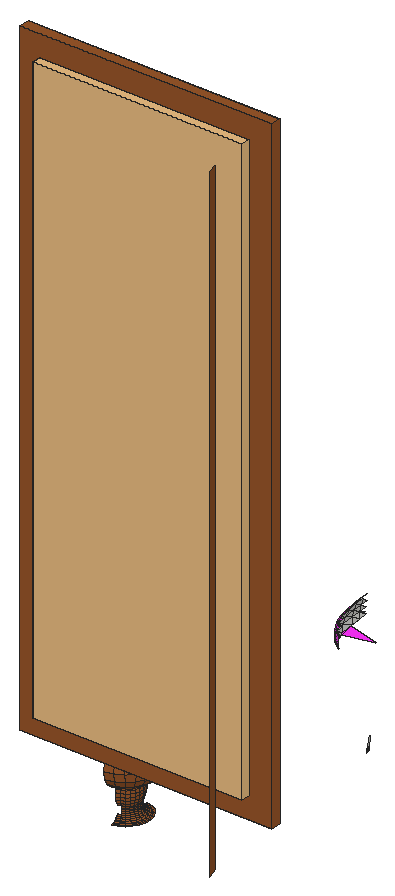
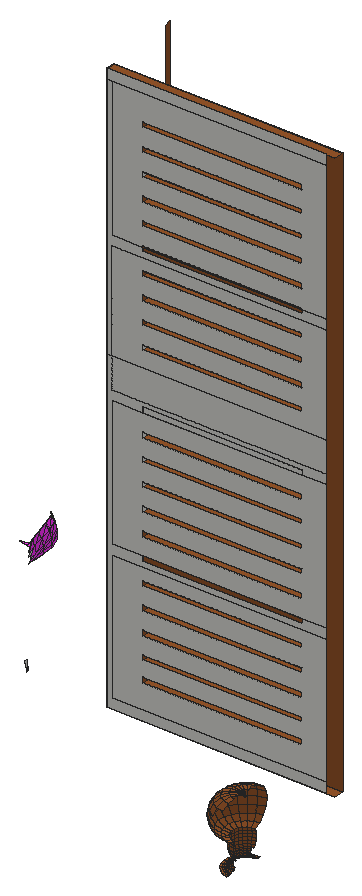
# SketchUp Ruby script. Lengths in inches.
U = 1.inch
M = Sketchup.active_model
def pt(a) = Geom::Point3d.new(a.map { |v| v * U })
def face(e, loops, mat)
  f = e.add_face(loops[0].map { |a| pt(a) })
  loops[1..].each { |l| e.add_face(l.map { |a| pt(a) }).erase! }
  f.material = f.back_material = mat if mat
  f
end
# faces: each face lists its corners as indices into pts; further lists are holes
def faces(e, pts, list, mat = nil) = list.each { |f| face(e, (f[0].is_a?(Array) ? f : [f]).map { |l| l.map { |i| pts[i] } }, mat) }
# xy, xz, yz: faces in a plane at the given z, y or x. An outline is a flat list of corners, or four numbers for a rectangle; further outlines are holes
def ring(l) = l.size == 4 ? [[l[0], l[1]], [l[2], l[1]], [l[2], l[3]], [l[0], l[3]]] : l.each_slice(2).to_a
def flat(e, list, mat, &to3) = list.each { |f| face(e, (f[0].is_a?(Array) ? f : [f]).map { |l| ring(l).map { |u, v| to3.(u, v) } }, mat) }
def xy(e, z, list, mat = nil) = flat(e, list, mat) { |x, y| [x, y, z] }
def xz(e, y, list, mat = nil) = flat(e, list, mat) { |x, z| [x, y, z] }
def yz(e, x, list, mat = nil) = flat(e, list, mat) { |y, z| [x, y, z] }
def lines(e, pts, list) = list.each { |a, b| e.add_line(pt(pts[a]), pt(pts[b])) }
# prism: a flat outline (further loops are holes) pulled along v
def prism(e, loops, v, mat = nil)
  f = face(e, loops, mat); d = Geom::Vector3d.new(v.map { |x| x * U })
  f.pushpull(f.normal.samedirection?(d) ? d.length : -d.length)
end
def box(e, o, s, mat = nil) = prism(e, [[o, [o[0] + s[0], o[1], o[2]], [o[0] + s[0], o[1] + s[1], o[2]], [o[0], o[1] + s[1], o[2]]]], [0, 0, s[2]], mat)
def at(x, y, z, deg = 0) = Geom::Transformation.translation(pt([x, y, z])) * Geom::Transformation.rotation(ORIGIN, Z_AXIS, deg.degrees)
def axes(o, x, y, z) = Geom::Transformation.new([*x, 0, *y, 0, *z, 0, *pt(o).to_a, 1])
def part(name) = M.definitions.add(name)
# library, detail: a bought-in or finely detailed component or shape, given as its bounding box
def library(name, o, s) = part(name).tap { |d| box(d.entities, o, s) }
def detail(e, o, s) = box(e.add_group.entities, o, s)
def put(e, d, t, mat = nil) = e.add_instance(d, t).tap { |i| i.material = mat if mat }
def group(e, t, mat = nil) = e.add_group.tap { |g| g.transformation = t; g.material = mat if mat }.entities
root = M.entities
M.materials.add("[Color K04]").color = [255, 50, 255]
M.materials.add("[Wood Cherry Original]").color = [152, 86, 42]
c1 = part("Group\#13")
detail(c1.entities,[0,0,0],[19.875,0.8125,55.92])
xy(root,6,[[161.3,47.97,161.84,48.11,161.78,48.25,161.28,48.12],[161.84,48.11,162.32,48.39,162.23,48.51,161.78,48.25],[162.32,48.39,162.72,48.78,162.6,48.87,162.23,48.51],[162.72,48.78,163,49.26,162.86,49.32,162.6,48.87],[163,49.26,163.15,49.8,163,49.82,162.86,49.32],
  [163.15,49.8,163.15,50.36,163,50.34,163,49.82],[163,50.34,163.15,50.36,163.01,50.9,162.87,50.84],[162.87,50.84,163.01,50.9,162.73,51.38,162.61,51.29],[162.61,51.29,162.73,51.38,162.34,51.78,162.24,51.66],[162.24,51.66,162.34,51.78,161.85,52.06,161.8,51.92],
  [161.8,51.92,161.85,52.06,161.32,52.21,161.3,52.06]],"[Wood Cherry Original]")
xy(root,13.08,[[154.9,45.11,178.85,46.11]],"[Wood Cherry Original]")
xy(root,16.73,[[158.4,45.11,175.02,46.11]],"[Wood Cherry Original]")
xy(root,17.26,[[158.4,45.11,175.02,46.11]],"[Wood Cherry Original]")
xy(root,18.83,[[158.4,45.11,175.02,46.11]],"[Wood Cherry Original]")
xy(root,19.33,[[158.4,45.11,175.02,46.11]],"[Wood Cherry Original]")
xy(root,21.15,[[158.4,45.11,175.02,46.11]],"[Wood Cherry Original]")
xy(root,21.65,[[158.4,45.11,175.02,46.11]],"[Wood Cherry Original]")
xy(root,23.48,[[158.4,45.11,175.02,46.11]],"[Wood Cherry Original]")
xy(root,23.98,[[158.4,45.11,175.02,46.11]],"[Wood Cherry Original]")
xy(root,25.8,[[158.4,45.11,175.02,46.11]],"[Wood Cherry Original]")
xy(root,26.3,[[158.4,45.11,175.02,46.11]],"[Wood Cherry Original]")
xy(root,28.125,[[158.4,45.11,175.02,46.11]],"[Wood Cherry Original]")
xy(root,28.625,[[158.4,45.11,175.02,46.11]],"[Wood Cherry Original]")
xy(root,30.45,[[158.4,45.11,175.02,46.11]],"[Wood Cherry Original]")
xy(root,30.95,[[158.4,45.11,175.02,46.11]],"[Wood Cherry Original]")
xy(root,32.78,[[158.4,45.11,175.02,46.11]],"[Wood Cherry Original]")
xy(root,33.28,[[158.4,45.11,175.02,46.11]],"[Wood Cherry Original]")
xy(root,35.1,[[158.4,45.11,175.02,46.11]],"[Wood Cherry Original]")
xy(root,35.6,[[158.4,45.11,175.02,46.11]])
xy(root,37.43,[[158.4,45.11,175.02,46.11]],"[Wood Cherry Original]")
xy(root,37.93,[[158.4,45.11,175.02,46.11]])
xy(root,39.75,[[158.4,45.11,175.02,46.11]],"[Wood Cherry Original]")
xy(root,40.25,[[158.4,45.11,175.02,46.11]])
xy(root,42.08,[[158.4,45.11,175.02,46.11]],"[Wood Cherry Original]")
xy(root,42.58,[[158.4,45.11,175.02,46.11]])
xy(root,47.97,[[158.4,45.11,175.02,46.11]],"[Wood Cherry Original]")
xy(root,48.47,[[158.4,45.11,175.02,46.11]])
xy(root,50.29,[[158.4,45.11,175.02,46.11]],"[Wood Cherry Original]")
xy(root,50.79,[[158.4,45.11,175.02,46.11]],"[Wood Cherry Original]")
xy(root,52.62,[[158.4,45.11,175.02,46.11]],"[Wood Cherry Original]")
xy(root,53.12,[[158.4,45.11,175.02,46.11]],"[Wood Cherry Original]")
xy(root,54.94,[[158.4,45.11,175.02,46.11]],"[Wood Cherry Original]")
xy(root,55.44,[[158.4,45.11,175.02,46.11]],"[Wood Cherry Original]")
xy(root,57.27,[[158.4,45.11,175.02,46.11]],"[Wood Cherry Original]")
xy(root,57.77,[[158.4,45.11,175.02,46.11]],"[Wood Cherry Original]")
xy(root,59.59,[[158.4,45.11,175.02,46.11]],"[Wood Cherry Original]")
xy(root,60.09,[[158.4,45.11,175.02,46.11]],"[Wood Cherry Original]")
xy(root,61.92,[[158.4,45.11,175.02,46.11]],"[Wood Cherry Original]")
xy(root,62.42,[[158.4,45.11,175.02,46.11]],"[Wood Cherry Original]")
xy(root,64.24,[[158.4,45.11,175.02,46.11]],"[Wood Cherry Original]")
xy(root,64.74,[[158.4,45.11,175.02,46.11]])
xy(root,66.57,[[158.4,45.11,175.02,46.11]],"[Wood Cherry Original]")
xy(root,67.07,[[158.4,45.11,175.02,46.11]])
xy(root,68.89,[[158.4,45.11,175.02,46.11]],"[Wood Cherry Original]")
xy(root,69.39,[[158.4,45.11,175.02,46.11]])
xy(root,73.08,[[154.9,45.11,178.85,46.11]],"[Wood Cherry Original]")
xz(root,45.11,[[[154.9,13.08,178.85,73.08],[158.4,16.73,175.02,69.39]],[158.4,17.26,175.02,18.83],[158.4,19.33,175.02,21.15],[158.4,21.65,175.02,23.48],[158.4,23.98,175.02,25.8],
  [158.4,26.3,175.02,28.125],[158.4,28.625,175.02,30.45],[158.4,30.95,175.02,32.78],[158.4,33.28,175.02,35.1],[158.4,35.6,175.02,37.43],
  [158.4,37.93,175.02,39.75],[158.4,40.25,175.02,42.08],[158.4,42.58,175.02,47.97],[158.4,48.47,175.02,50.29],[158.4,50.79,175.02,52.62],
  [158.4,53.12,175.02,54.94],[158.4,55.44,175.02,57.27],[158.4,57.77,175.02,59.59],[158.4,60.09,175.02,61.92],[158.4,62.42,175.02,64.24],
  [158.4,64.74,175.02,66.57],[158.4,67.07,175.02,68.89]],"[Wood Cherry Original]")
xz(root,46.11,[[155.9,13.08,178.85,13.08,178.85,46.26,178.35,46.26,178.35,43.08,155.9,43.08,155.9,42.08,158.4,42.08,158.4,42.58,175.02,42.58,175.02,42.08,178.35,42.08,178.35,28.58,175.02,28.58,175.02,28.125,158.4,28.125,158.4,28.58,155.9,28.58,155.9,27.58,178.35,27.58,178.35,14.08,155.9,14.08],[[155.9,13.08,155.9,43.08,178.35,43.08,178.35,46.26,178.85,46.26,178.85,13.08],[158.4,16.73,175.02,17.26],[158.4,42.08,175.02,42.58],[158.4,39.75,175.02,40.25],[158.4,37.43,175.02,37.93],[158.4,35.1,175.02,35.6],[158.4,32.78,175.02,33.28],[158.4,30.45,175.02,30.95],[158.4,28.125,175.02,28.625],[158.4,25.8,175.02,26.3],[158.4,23.48,175.02,23.98],[158.4,18.83,175.02,19.33],[158.4,21.15,175.02,21.65]],[158.4,42.08,175.02,42.58],[155.9,43.08,178.35,46.26],[178.35,46.26,178.85,46.26,178.85,72.08,178.35,72.08,178.35,57.58,175.02,57.58,175.02,57.27,158.4,57.27,158.4,57.58,155.9,57.58,155.9,56.58,178.35,56.58],
  [[155.9,46.26,178.35,56.58],[158.4,47.97,175.02,48.47],[158.4,50.29,175.02,50.79],[158.4,52.62,175.02,53.12],[158.4,54.94,175.02,55.44]],[[178.35,46.26,178.35,56.58,155.9,56.58,155.9,72.08,178.85,72.08,178.85,46.26],[158.4,68.89,175.02,69.39],[158.4,66.57,175.02,67.07],[158.4,64.24,175.02,64.74],[158.4,61.92,175.02,62.42],[158.4,59.59,175.02,60.09],[158.4,57.27,175.02,57.77]],[155.9,72.08,178.85,73.08]])
xz(root,46.11,[[158.4,28.125,175.02,28.58],[158.4,57.27,175.02,57.58]],"[Wood Cherry Original]")
yz(root,162.22,[[49.93,6.79,50.24,6.94]],"[Wood Cherry Original]")
yz(root,175.02,[[45.11,32.78,46.11,33.28],[45.11,35.1,46.11,35.6],[45.11,37.43,46.11,37.93],[45.11,39.75,46.11,40.25],[45.11,42.08,46.11,42.58],
  [45.11,47.97,46.11,48.47],[45.11,64.24,46.11,64.74]])
yz(root,175.02,[[45.11,16.73,46.11,17.26],[45.11,18.83,46.11,19.33],[45.11,21.15,46.11,21.65],[45.11,23.48,46.11,23.98],[45.11,25.8,46.11,26.3],
  [45.11,28.125,46.11,28.625],[45.11,30.45,46.11,30.95],[45.11,50.29,46.11,50.79],[45.11,52.62,46.11,53.12],[45.11,54.94,46.11,55.44],
  [45.11,57.27,46.11,57.77],[45.11,59.59,46.11,60.09],[45.11,61.92,46.11,62.42],[45.11,66.57,46.11,67.07],[45.11,68.89,46.11,69.39]],"[Wood Cherry Original]")
yz(root,178.85,[[45.11,13.08,46.11,73.08]],"[Wood Cherry Original]")
p = [[161.26,48.26,6.03],[161.28,48.12,6],[161.78,48.25,6],[161.73,48.39,6.03],[162.23,48.51,6],[162.14,48.625,6.03],
  [161.24,48.4,6.08],[161.67,48.52,6.08],[162.06,48.74,6.08],[162.6,48.87,6],[162.48,48.96,6.03],[162.37,49.05,6.08],
  [162.86,49.32,6],[162.72,49.375,6.03],[162.59,49.43,6.08],[163,49.82,6],[162.85,49.84,6.03],[162.71,49.86,6.08],
  [162.85,50.32,6.03],[162.71,50.3,6.08],[163,50.34,6],[162.73,50.78,6.03],[162.6,50.73,6.08],[162.87,50.84,6],
  [162.49,51.2,6.03],[162.38,51.11,6.08],[162.61,51.29,6],[162.15,51.54,6.03],[162.07,51.43,6.08],[162.24,51.66,6],
  [161.74,51.78,6.03],[161.68,51.65,6.08],[161.8,51.92,6],[161.28,51.91,6.03],[161.26,51.77,6.08],[161.3,52.06,6],
  [161.23,48.53,6.16],[161.62,48.64,6.16],[161.98,48.84,6.16],[162.27,49.13,6.16],[162.47,49.48,6.16],[162.58,49.875,6.16],
  [162.58,50.29,6.16],[162.48,50.68,6.16],[162.27,51.04,6.16],[161.99,51.33,6.16],[161.63,51.53,6.16],[161.24,51.64,6.16],
  [161.21,48.65,6.25],[161.58,48.74,6.25],[161.91,48.93,6.25],[162.18,49.2,6.25],[162.37,49.53,6.25],[162.47,49.89,6.25],
  [162.47,50.27,6.25],[162.37,50.64,6.25],[162.18,50.97,6.25],[161.92,51.23,6.25],[161.59,51.43,6.25],[161.22,51.52,6.25],
  [161.2,48.74,6.37],[161.54,48.83,6.37],[161.85,49.01,6.37],[162.1,49.26,6.37],[162.28,49.5625,6.37],[162.37,49.91,6.37],
  [162.37,50.26,6.37],[162.28,50.6,6.37],[162.11,50.91,6.37],[161.86,51.16,6.37],[161.55,51.34,6.37],[161.21,51.43,6.37],
  [161.19,48.82,6.5],[161.51,48.9,6.5],[161.8,49.07,6.5],[162.04,49.3,6.5],[162.21,49.59,6.5],[162.3,49.92,6.5],
  [162.3,50.25,6.5],[162.21,50.57,6.5],[162.05,50.86,6.5],[161.8125,51.1,6.5],[161.52,51.27,6.5],[161.2,51.35,6.5],
  [161.49,48.95,6.64],[161.77,49.11,6.64],[162,49.34,6.64],[162.16,49.61,6.64],[162.24,49.92,6.64],[162.25,50.24,6.64],
  [162.16,50.55,6.64],[162,50.83,6.64],[161.78,51.06,6.64],[161.5,51.22,6.64],[161.48,48.98,6.79],[161.76,49.13,6.79],
  [161.98,49.35,6.79],[162.14,49.62,6.79],[162.22,49.93,6.79],[162.22,50.24,6.79],[162.14,50.54,6.79],[161.98,50.82,6.79],
  [161.76,51.04,6.79],[161.49,51.2,6.79],[161.48,48.97,6.94],[161.76,49.13,6.94],[161.98,49.35,6.94],[162.14,49.62,6.94],
  [162.22,49.93,6.94],[162.22,50.24,6.94],[162.14,50.54,6.94],[161.98,50.82,6.94],[161.76,51.04,6.94],[161.49,51.2,6.94],
  [161.49,48.95,7.09],[161.77,49.11,7.09],[162,49.34,7.09],[162.16,49.61,7.09],[162.25,49.92,7.09],[162.25,50.24,7.09],
  [162.16,50.55,7.09],[162.01,50.83,7.09],[161.78,51.06,7.09],[161.5,51.22,7.09],[161.51,48.9,7.23],[161.8,49.07,7.23],
  [162.04,49.3,7.23],[162.21,49.59,7.23],[162.3,49.92,7.23],[162.3,50.25,7.23],[162.21,50.57,7.23],[162.05,50.86,7.23],
  [161.8125,51.1,7.23],[161.52,51.27,7.23],[161.19,51.3,7.09],[161.2,51.36,7.23],[161.2,48.71,7.51],[161.19,48.82,7.23],
  [161.56,48.8,7.51],[161.87,48.98,7.51],[162.13,49.24,7.51],[162.3125,49.55,7.51],[162.41,49.9,7.51],[162.41,50.26,7.51],
  [162.32,50.61,7.51],[162.14,50.93,7.51],[161.88,51.1875,7.51],[161.57,51.37,7.51],[161.22,51.47,7.51],[161.21,48.63,7.8],
  [161.58,48.73,7.8],[161.92,48.92,7.8],[162.1875,49.1875,7.8],[162.38,49.52,7.8],[162.48,49.89,7.8],[162.48,50.27,7.8],
  [162.39,50.64,7.8],[162.2,50.98,7.8],[161.93,51.25,7.8],[161.59,51.44,7.8],[161.23,51.54,7.8],[161.22,48.59,8.1],
  [161.6,48.69,8.1],[161.94,48.89,8.1],[162.22,49.16,8.1],[162.42,49.5,8.1],[162.52,49.88,8.1],[162.52,50.28,8.1],
  [162.42,50.66,8.1],[162.23,51,8.1],[161.95,51.28,8.1],[161.61,51.48,8.1],[161.23,51.58,8.1],[161.22,48.59,8.4],
  [161.6,48.69,8.4],[161.94,48.89,8.4],[162.22,49.16,8.4],[162.42,49.5,8.4],[162.52,49.88,8.4],[162.53,50.28,8.4],
  [162.43,50.66,8.4],[162.23,51,8.4],[161.95,51.28,8.4],[161.61,51.48,8.4],[161.23,51.58,8.4],[161.22,48.62,8.7],
  [161.59,48.72,8.7],[161.92,48.91,8.7],[162.2,49.18,8.7],[162.39,49.52,8.7],[162.49,49.89,8.7],[162.49,50.27,8.7],
  [162.39,50.65,8.7],[162.2,50.98,8.7],[161.93,51.25,8.7],[161.6,51.45,8.7],[161.23,51.55,8.7],[161.21,48.69,8.99],
  [161.5625,48.79,8.99],[161.88,48.97,8.99],[162.14,49.23,8.99],[162.32,49.54,8.99],[162.42,49.9,8.99],[162.42,50.27,8.99],
  [162.33,50.62,8.99],[162.15,50.9375,8.99],[161.89,51.2,8.99],[161.57,51.38,8.99],[161.22,51.48,8.99],[161.3,48,9.21],
  [161.83,48.14,9.21],[162.3,48.41,9.21],[162.7,48.8,9.21],[162.97,49.27,9.21],[163.12,49.8,9.21],[163.12,50.35,9.21],
  [162.98,50.89,9.21],[162.71,51.36,9.21],[162.32,51.75,9.21],[161.84,52.03,9.21],[161.3125,52.18,9.21],[161.37,47.42,9.66],
  [162.05,47.6,9.66],[162.66,47.95,9.66],[163.15,48.44,9.66],[163.51,49.05,9.66],[163.69,49.73,9.66],[163.69,50.43,9.66],
  [163.51,51.11,9.66],[163.17,51.71,9.66],[162.67,52.21,9.66],[162.07,52.57,9.66],[161.39,52.75,9.66],[161.42,47.04,10.28],
  [162.19,47.25,10.28],[162.89,47.65,10.28],[163.45,48.21,10.28],[163.86,48.9,10.28],[164.07,49.68,10.28],[164.07,50.48,10.28],
  [163.87,51.25,10.28],[163.47,51.94,10.28],[162.9,52.51,10.28],[162.21,52.92,10.28],[161.43,46.91,11],[162.24,47.125,11],
  [162.97,47.54,11],[163.56,48.13,11],[163.98,48.85,11],[164.2,49.66,11],[164.2,50.49,11],[163.99,51.3,11],
  [163.57,52.03,11],[162.99,52.62,11],[161.42,47.04,11.72],[162.19,47.25,11.72],[162.89,47.65,11.72],[163.45,48.21,11.72],
  [163.86,48.9,11.72],[164.07,49.68,11.72],[164.07,50.48,11.72],[163.87,51.25,11.72],[163.47,51.94,11.72],[162.9,52.51,11.72],
  [161.37,47.42,12.34],[162.05,47.6,12.34],[162.66,47.95,12.34],[163.15,48.44,12.34],[163.51,49.05,12.34],[163.69,49.73,12.34],
  [163.69,50.43,12.34],[163.51,51.11,12.34],[163.17,51.71,12.34],[162.67,52.21,12.34],[162.21,52.92,11.72],[162.07,52.57,12.34],
  [161.3,48,12.79],[161.83,48.14,12.79],[162.3,48.41,12.79],[162.7,48.8,12.79],[162.97,49.27,12.79],[163.12,49.8,12.79],
  [163.12,50.35,12.79],[162.98,50.89,12.79],[162.71,51.36,12.79],[162.32,51.75,12.79],[161.84,52.03,12.79],[161.39,52.75,12.34],
  [161.3125,52.18,12.79],[161.03,50.09,12.67],[161.56,49.68,12.97],[161.65,49.83,12.97],[161.69,50,12.97],[161.69,50.17,12.97],
  [161.65,50.34,12.97],[161.5625,50.49,12.97],[161.21,48.69,13.01],[161.5625,48.79,13.01],[161.88,48.97,13.01],[162.14,49.23,13.01],
  [162.32,49.54,13.01],[162.42,49.9,13.01],[162.42,50.27,13.01],[162.33,50.62,13.01],[162.15,50.9375,13.01],[161.89,51.2,13.01],
  [161.57,51.38,13.01],[161.22,51.48,13.01],[161.28,49.47,12.97],[161.43,49.55,12.97],[161.4375,50.62,12.97],[161.29,50.71,12.97],
  [179.45,37.53,13.08],[179.8,36.6,13.08],[179.8,36.6,73.08],[179.45,37.53,73.08],[179.45,37.53,46.26],[182.43,51.92,17.77],
  [182.35,52.19,17.8125],[182.35,52.2,17.86],[182.4,52.07,18],[182.44,51.93,18.14],[182.34,52.25,17.82],[182.35,52.24,18.01],
  [182.3,52.48,18.99],[182.4,52.09,18.17],[182.4,52.16,18.88],[182.35,52.23,18.19],[182.13,48.48,28.67],[182.22,48.5,28.59],
  [182.89,47.98,28.59],[181.67,49.76,28.67],[181.75,49.77,28.59],[181.58,51.11,28.65],[181.5,51.1,28.73],[184.52,50.36,28.59],
  [182.13,48.48,28.96],[182.87,47.89,28.67],[182.87,47.89,28.96],[182.27,48.54,28.72],[182.26,48.59,29.63],[182.9,48.03,29.63],
  [181.67,49.76,28.96],[181.81,49.78,28.72],[181.79,49.8125,29.53],[181.5,51.1,28.96],[181.63,51.12,28.78],[181.375,52.2,28.96],
  [181.375,52.2,28.74],[181.45,52.22,28.66],[181.48,52.21,29.37],[181.51,52.23,28.79],[181.39,53.13,28.71],[181.625,51.09,29.45],
  [181.26,53.1,28.875],[181.49,51.08,29.47],[181.34,52.1875,29.38],[182.86,47.9,29.65],[182.14,48.51,29.65],[181.66,49.78,29.55],
  [181.23,53.09,29.34],[181.45,52.23,29.97],[181.59,52.25,29.9375],[181.37,53.11,29.33],[181.64,51.15,30.09],[181.77,51.17,30.05],
  [182.38,48.68,30.28],[181.98,49.86,30.17],[181.85,49.83,30.23],[182.9,48.04,30.32],[182.27,48.6,30.32],[182.93,48.17,30.28],
  [181.93,51.25,30.58],[181.72,52.32,30.46],[181.3,53.11,29.89],[181.6,52.3,30.55],[181.4375,53.13,29.86],[181.82,51.23,30.68],
  [182.16,49.97,30.79],[182.25,49.98,30.67],[182.51,48.74,30.9],[182.6,48.79,30.78],[182.93,48.29,30.9],[181.9,51.25,30.66],
  [181.67,52.3125,30.53],[181.47,53.14,30.46],[182.23,49.98,30.75],[182.58,48.78,30.86]]
faces(root,p,[[0,1,2,3],[3,2,4,5],[6,0,3,7],[7,3,5,8],[5,4,9,10],[8,5,10,11],[10,9,12,13],[11,10,13,14],
  [13,12,15,16],[14,13,16,17],[17,16,18,19],[16,15,20,18],[19,18,21,22],[18,20,23,21],[22,21,24,25],[21,23,26,24],
  [25,24,27,28],[24,26,29,27],[28,27,30,31],[27,29,32,30],[31,30,33,34],[30,32,35,33],[36,6,7,37],[37,7,8,38],
  [38,8,11,39],[39,11,14,40],[40,14,17,41],[41,17,19,42],[42,19,22,43],[43,22,25,44],[44,25,28,45],[45,28,31,46],
  [46,31,34,47],[48,36,37,49],[49,37,38,50],[50,38,39,51],[51,39,40,52],[52,40,41,53],[53,41,42,54],[54,42,43,55],
  [55,43,44,56],[56,44,45,57],[57,45,46,58],[58,46,47,59],[60,48,49,61],[61,49,50,62],[62,50,51,63],[63,51,52,64],
  [64,52,53,65],[65,53,54,66],[66,54,55,67],[67,55,56,68],[68,56,57,69],[69,57,58,70],[70,58,59,71],[72,60,61,73],
  [73,61,62,74],[74,62,63,75],[75,63,64,76],[76,64,65,77],[77,65,66,78],[78,66,67,79],[79,67,68,80],[80,68,69,81],
  [81,69,70,82],[82,70,71,83],[84,73,74,85],[85,74,75,86],[86,75,76,87],[87,76,77,88],[88,77,78,89],[89,78,79,90],
  [90,79,80,91],[91,80,81,92],[92,81,82,93],[94,84,85,95],[95,85,86,96],[96,86,87,97],[97,87,88,98],[98,88,89,99],
  [99,89,90,100],[100,90,91,101],[101,91,92,102],[102,92,93,103],[104,94,95,105],[105,95,96,106],[106,96,97,107],[107,97,98,108],
  [109,99,100,110],[110,100,101,111],[111,101,102,112],[112,102,103,113],[114,104,105,115],[115,105,106,116],[116,106,107,117],[117,107,108,118],
  [118,108,109,119],[119,109,110,120],[120,110,111,121],[121,111,112,122],[122,112,113,123],[124,114,115,125],[125,115,116,126],[126,116,117,127],
  [127,117,118,128],[128,118,119,129],[129,119,120,130],[130,120,121,131],[131,121,122,132],[132,122,123,133],[133,123,134,135],[136,137,124,138],
  [138,124,125,139],[139,125,126,140],[140,126,127,141],[141,127,128,142],[142,128,129,143],[143,129,130,144],[144,130,131,145],[145,131,132,146],
  [146,132,133,147],[147,133,135,148],[149,136,138,150],[150,138,139,151],[151,139,140,152],[152,140,141,153],[153,141,142,154],[154,142,143,155],
  [155,143,144,156],[156,144,145,157],[157,145,146,158],[158,146,147,159],[159,147,148,160],[161,149,150,162],[162,150,151,163],[163,151,152,164],
  [164,152,153,165],[165,153,154,166],[166,154,155,167],[167,155,156,168],[168,156,157,169],[169,157,158,170],[170,158,159,171],[171,159,160,172],
  [173,161,162,174],[174,162,163,175],[175,163,164,176],[176,164,165,177],[177,165,166,178],[178,166,167,179],[179,167,168,180],[180,168,169,181],
  [181,169,170,182],[182,170,171,183],[183,171,172,184],[185,173,174,186],[186,174,175,187],[187,175,176,188],[188,176,177,189],[189,177,178,190],
  [190,178,179,191],[191,179,180,192],[192,180,181,193],[193,181,182,194],[194,182,183,195],[195,183,184,196],[197,185,186,198],[198,186,187,199],
  [199,187,188,200],[200,188,189,201],[201,189,190,202],[202,190,191,203],[203,191,192,204],[204,192,193,205],[205,193,194,206],[206,194,195,207],
  [207,195,196,208],[209,197,198,210],[210,198,199,211],[211,199,200,212],[212,200,201,213],[213,201,202,214],[214,202,203,215],[215,203,204,216],
  [216,204,205,217],[217,205,206,218],[218,206,207,219],[219,207,208,220],[221,209,210,222],[222,210,211,223],[223,211,212,224],[224,212,213,225],
  [225,213,214,226],[226,214,215,227],[227,215,216,228],[228,216,217,229],[229,217,218,230],[230,218,219,231],[231,219,220,232],[233,221,222,234],
  [234,222,223,235],[235,223,224,236],[236,224,225,237],[237,225,226,238],[238,226,227,239],[239,227,228,240],[240,228,229,241],[241,229,230,242],
  [242,230,231,243],[244,233,234,245],[245,234,235,246],[246,235,236,247],[247,236,237,248],[248,237,238,249],[249,238,239,250],[250,239,240,251],
  [251,240,241,252],[252,241,242,253],[254,244,245,255],[255,245,246,256],[256,246,247,257],[257,247,248,258],[258,248,249,259],[259,249,250,260],
  [260,250,251,261],[261,251,252,262],[262,252,253,263],[264,254,255,265],[265,255,256,266],[266,256,257,267],[267,257,258,268],[268,258,259,269],
  [269,259,260,270],[270,260,261,271],[271,261,262,272],[272,262,263,273],[273,263,274,275],[276,264,265,277],[277,265,266,278],[278,266,267,279],
  [279,267,268,280],[280,268,269,281],[281,269,270,282],[282,270,271,283],[283,271,272,284],[284,272,273,285],[285,273,275,286],[286,275,287,288],
  [289,290,291],[289,291,292],[289,292,293],[289,293,294],[289,294,295],[296,276,277,297],[297,277,278,298],[298,278,279,299],
  [299,279,280,300],[300,280,281,301],[301,281,282,302],[302,282,283,303],[303,283,284,304],[304,284,285,305],[305,285,286,306],[306,286,288,307],
  [308,297,298,309],[309,298,299,290],[290,299,300,291],[291,300,301,292],[292,301,302,293],[293,302,303,294],[294,303,304,295],[295,304,305,310],
  [310,305,306,311],[312,313,314,315,316]],"[Wood Cherry Original]")
faces(root,p,[[317,318,319,320,321],[322,323,319],[324,323,319,320,325,326],[320,319,323,327,325],[339,340,341],[340,339,343],[343,344,340],[344,343,346],
  [350,351,352],[346,353,344],[353,346,351],[351,350,353],[362,350,363],[365,353,350],[350,362,365],[366,340,344],
  [344,367,366],[367,344,353],[353,365,367],[340,366,371],[372,365,362],[362,373,372],[373,362,376],[379,367,365],
  [365,372,379],[381,366,367],[367,379,381],[383,384,375],[383,372,373],[373,384,383],[385,375,384],[386,379,372],
  [372,383,386],[375,377,383],[379,386,387],[387,381,379],[377,378,386],[386,383,377],[378,380,387],[387,386,378]])
faces(root,p,[[328,329,330],[329,328,331],[331,332,329],[333,332,331,334],[335,332,333],[336,328,337,338],[342,331,328,336],[345,334,331,342],
  [347,348,334,345],[349,333,334,348],[354,347,355,356],[336,338,357],[357,358,336],[342,336,358],[358,359,342],[345,342,359],
  [359,355,345],[347,345,355],[360,356,361],[356,355,364],[364,361,356],[355,359,368],[368,364,355],[369,370,358],
  [359,358,370],[370,368,359],[374,361,375],[361,364,377],[377,375,361],[364,368,378],[378,377,364],[368,370,380],
  [380,378,368],[382,380,370]],"[Color K04]")
put(root,c1,at(156.78,44.3,15.1),"[Wood Cherry Original]")
